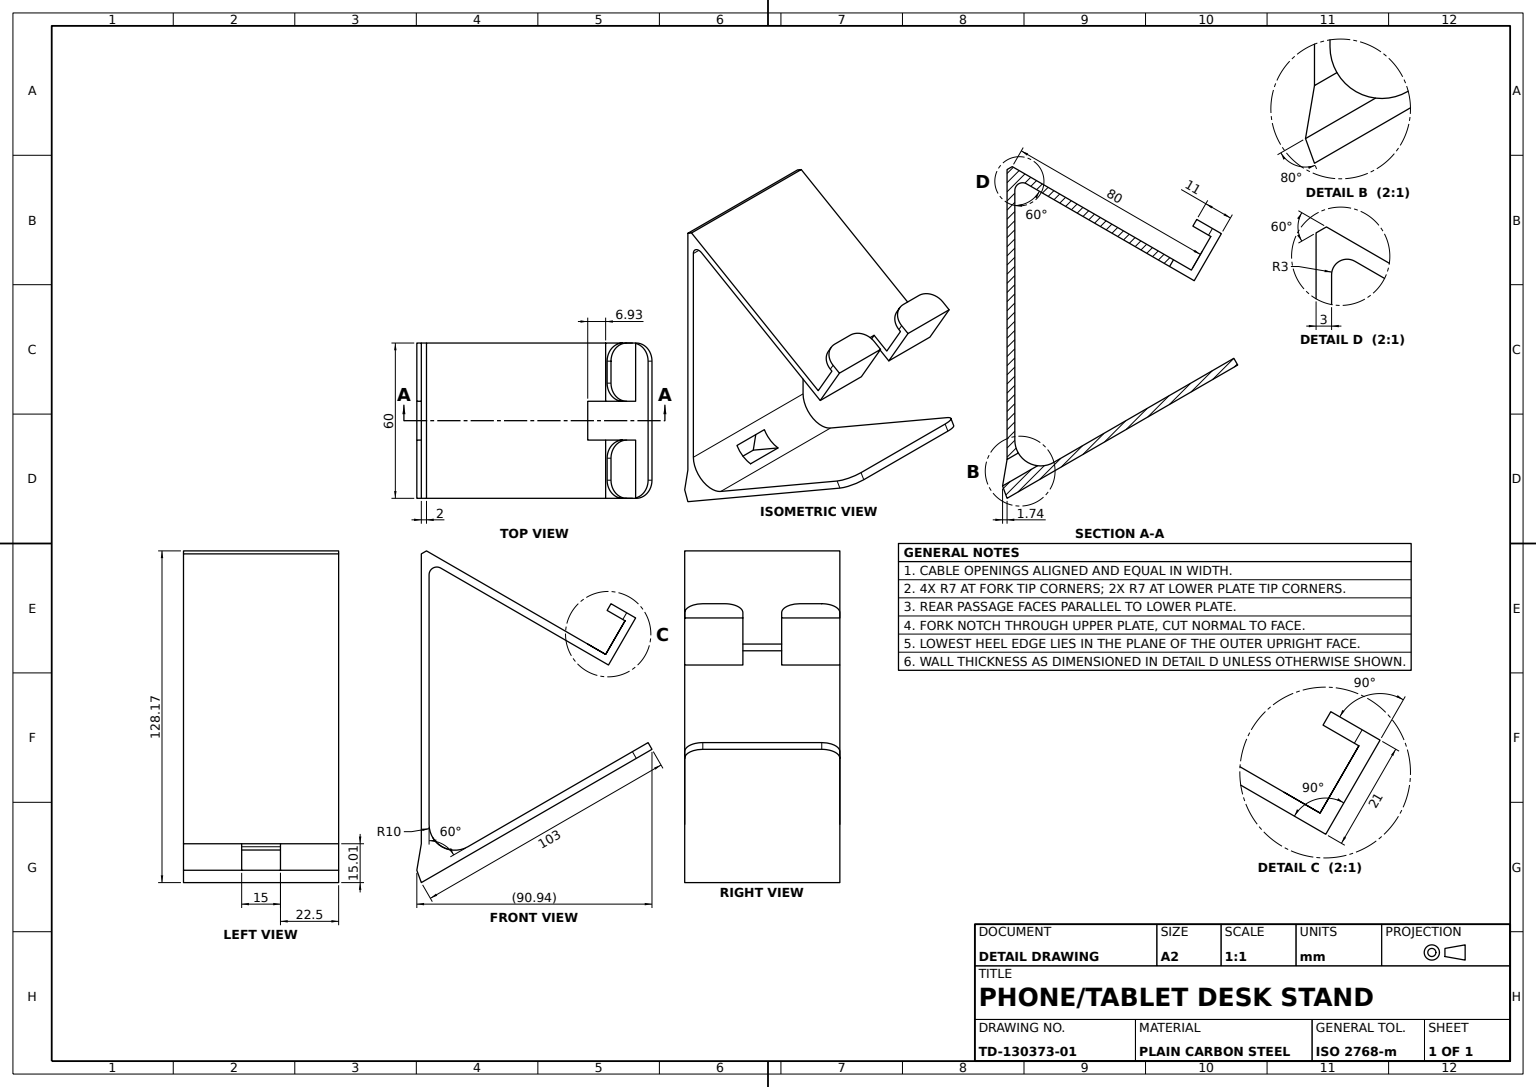
ISO-10303-21;
HEADER;
FILE_DESCRIPTION((''),'2;1');
FILE_NAME('','',(''),(''),'','','');
FILE_SCHEMA(('AUTOMOTIVE_DESIGN'));
ENDSEC;
DATA;
#1=APPLICATION_CONTEXT('');
#2=PRODUCT_CONTEXT('',#1,'mechanical');
#3=PRODUCT('','','',(#2));
#4=PRODUCT_DEFINITION_FORMATION('','',#3);
#5=PRODUCT_DEFINITION_CONTEXT('',#1,'design');
#6=PRODUCT_DEFINITION('','',#4,#5);
#7=PRODUCT_DEFINITION_SHAPE('','',#6);
#8=(LENGTH_UNIT()NAMED_UNIT(*)SI_UNIT(.MILLI.,.METRE.));
#9=(NAMED_UNIT(*)PLANE_ANGLE_UNIT()SI_UNIT($,.RADIAN.));
#10=(NAMED_UNIT(*)SI_UNIT($,.STERADIAN.)SOLID_ANGLE_UNIT());
#11=UNCERTAINTY_MEASURE_WITH_UNIT(LENGTH_MEASURE(1.E-05),#8,'distance_accuracy_value','');
#12=(GEOMETRIC_REPRESENTATION_CONTEXT(3)GLOBAL_UNCERTAINTY_ASSIGNED_CONTEXT((#11))GLOBAL_UNIT_ASSIGNED_CONTEXT((#8,#9,#10))REPRESENTATION_CONTEXT('',''));
#13=CARTESIAN_POINT('',(102.118365,2.,-7.5));
#14=VERTEX_POINT('',#13);
#15=CARTESIAN_POINT('',(86.48334,2.,-7.5));
#16=VERTEX_POINT('',#15);
#17=CARTESIAN_POINT('',(103.,2.,-7.5));
#18=DIRECTION('',(-1.,0.,0.));
#19=VECTOR('',#18,1000.);
#20=LINE('',#17,#19);
#21=EDGE_CURVE('',#14,#16,#20,.T.);
#22=ORIENTED_EDGE('',*,*,#21,.F.);
#23=CARTESIAN_POINT('',(95.494447,10.,-7.5));
#24=VERTEX_POINT('',#23);
#25=DIRECTION('',(-0.637752207,0.7702416,0.));
#26=VECTOR('',#25,1000.);
#27=LINE('',#23,#26);
#28=EDGE_CURVE('',#14,#24,#27,.T.);
#29=ORIENTED_EDGE('',*,*,#28,.T.);
#30=CARTESIAN_POINT('',(90.48334,10.,-7.5));
#31=VERTEX_POINT('',#30);
#32=CARTESIAN_POINT('',(103.,10.,-7.5));
#33=LINE('',#32,#19);
#34=EDGE_CURVE('',#24,#31,#33,.T.);
#35=ORIENTED_EDGE('',*,*,#34,.T.);
#36=CARTESIAN_POINT('',(80.48334,10.,-7.5));
#37=DIRECTION('',(0.,0.,-1.));
#38=DIRECTION('',(1.,0.,0.));
#39=AXIS2_PLACEMENT_3D('',#36,#37,#38);
#40=CIRCLE('',#39,10.);
#41=EDGE_CURVE('',#31,#16,#40,.T.);
#42=ORIENTED_EDGE('',*,*,#41,.T.);
#43=EDGE_LOOP('',(#22,#29,#35,#42));
#44=FACE_OUTER_BOUND('',#43,.T.);
#45=DIRECTION('',(0.,0.,1.));
#46=AXIS2_PLACEMENT_3D('',#17,#45,#38);
#47=PLANE('',#46);
#48=ADVANCED_FACE('',(#44),#47,.T.);
#49=CARTESIAN_POINT('',(-14.406388,53.646171,-23.));
#50=VERTEX_POINT('',#49);
#51=CARTESIAN_POINT('',(-17.906388,47.583993,-30.));
#52=VERTEX_POINT('',#51);
#53=CARTESIAN_POINT('',(-17.906388,47.583993,-23.));
#54=DIRECTION('',(-0.866025404,0.5,0.));
#55=DIRECTION('',(0.5,0.866025404,0.));
#56=AXIS2_PLACEMENT_3D('',#53,#54,#55);
#57=CIRCLE('',#56,7.);
#58=EDGE_CURVE('',#50,#52,#57,.T.);
#59=ORIENTED_EDGE('',*,*,#58,.F.);
#60=CARTESIAN_POINT('',(-11.808312,52.146171,-23.));
#61=VERTEX_POINT('',#60);
#62=VECTOR('',#54,1000.);
#63=LINE('',#49,#62);
#64=EDGE_CURVE('',#61,#50,#63,.T.);
#65=ORIENTED_EDGE('',*,*,#64,.F.);
#66=CARTESIAN_POINT('',(-15.308312,46.083993,-30.));
#67=VERTEX_POINT('',#66);
#68=CARTESIAN_POINT('',(-15.308312,46.083993,-23.));
#69=DIRECTION('',(0.866025404,-0.5,0.));
#70=DIRECTION('',(-0.5,-0.866025404,0.));
#71=AXIS2_PLACEMENT_3D('',#68,#69,#70);
#72=CIRCLE('',#71,7.);
#73=EDGE_CURVE('',#67,#61,#72,.T.);
#74=ORIENTED_EDGE('',*,*,#73,.F.);
#75=CARTESIAN_POINT('',(2.878222,35.583993,-30.));
#76=VECTOR('',#69,1000.);
#77=LINE('',#75,#76);
#78=EDGE_CURVE('',#52,#67,#77,.T.);
#79=ORIENTED_EDGE('',*,*,#78,.F.);
#80=EDGE_LOOP('',(#59,#65,#74,#79));
#81=FACE_OUTER_BOUND('',#80,.T.);
#82=AXIS2_PLACEMENT_3D('',#53,#54,#70);
#83=CYLINDRICAL_SURFACE('',#82,7.);
#84=ADVANCED_FACE('',(#81),#83,.T.);
#85=CARTESIAN_POINT('',(0.,0.,23.));
#86=VERTEX_POINT('',#85);
#87=CARTESIAN_POINT('',(7.,0.,30.));
#88=VERTEX_POINT('',#87);
#89=CARTESIAN_POINT('',(7.,0.,23.));
#90=DIRECTION('',(0.,1.,0.));
#91=AXIS2_PLACEMENT_3D('',#89,#90,#37);
#92=CIRCLE('',#91,7.);
#93=EDGE_CURVE('',#86,#88,#92,.T.);
#94=ORIENTED_EDGE('',*,*,#93,.F.);
#95=CARTESIAN_POINT('',(0.,-3.,23.));
#96=VERTEX_POINT('',#95);
#97=VECTOR('',#90,1000.);
#98=LINE('',#85,#97);
#99=EDGE_CURVE('',#96,#86,#98,.T.);
#100=ORIENTED_EDGE('',*,*,#99,.F.);
#101=CARTESIAN_POINT('',(7.,-3.,30.));
#102=VERTEX_POINT('',#101);
#103=CARTESIAN_POINT('',(7.,-3.,23.));
#104=DIRECTION('',(0.,-1.,0.));
#105=AXIS2_PLACEMENT_3D('',#103,#104,#18);
#106=CIRCLE('',#105,7.);
#107=EDGE_CURVE('',#102,#96,#106,.T.);
#108=ORIENTED_EDGE('',*,*,#107,.F.);
#109=VECTOR('',#104,1000.);
#110=LINE('',#101,#109);
#111=EDGE_CURVE('',#88,#102,#110,.T.);
#112=ORIENTED_EDGE('',*,*,#111,.F.);
#113=EDGE_LOOP('',(#94,#100,#108,#112));
#114=FACE_OUTER_BOUND('',#113,.T.);
#115=CARTESIAN_POINT('',(7.,97.,23.));
#116=AXIS2_PLACEMENT_3D('',#115,#90,#45);
#117=CYLINDRICAL_SURFACE('',#116,7.);
#118=ADVANCED_FACE('',(#114),#117,.T.);
#119=CARTESIAN_POINT('',(103.,-3.,30.));
#120=VERTEX_POINT('',#119);
#121=CARTESIAN_POINT('',(102.118365,2.,30.));
#122=VERTEX_POINT('',#121);
#123=DIRECTION('',(-0.173648178,0.984807753,0.));
#124=VECTOR('',#123,1000.);
#125=LINE('',#119,#124);
#126=EDGE_CURVE('',#120,#122,#125,.T.);
#127=ORIENTED_EDGE('',*,*,#126,.F.);
#128=CARTESIAN_POINT('',(103.,-3.,-30.));
#129=VERTEX_POINT('',#128);
#130=VECTOR('',#37,1000.);
#131=LINE('',#119,#130);
#132=EDGE_CURVE('',#120,#129,#131,.T.);
#133=ORIENTED_EDGE('',*,*,#132,.T.);
#134=CARTESIAN_POINT('',(102.118365,2.,-30.));
#135=VERTEX_POINT('',#134);
#136=LINE('',#128,#124);
#137=EDGE_CURVE('',#129,#135,#136,.T.);
#138=ORIENTED_EDGE('',*,*,#137,.T.);
#139=LINE('',#121,#130);
#140=EDGE_CURVE('',#14,#135,#139,.T.);
#141=ORIENTED_EDGE('',*,*,#140,.F.);
#142=CARTESIAN_POINT('',(102.118365,2.,7.5));
#143=VERTEX_POINT('',#142);
#144=EDGE_CURVE('',#143,#14,#139,.T.);
#145=ORIENTED_EDGE('',*,*,#144,.F.);
#146=EDGE_CURVE('',#122,#143,#139,.T.);
#147=ORIENTED_EDGE('',*,*,#146,.F.);
#148=EDGE_LOOP('',(#127,#133,#138,#141,#145,#147));
#149=FACE_OUTER_BOUND('',#148,.T.);
#150=DIRECTION('',(-0.984807753,-0.173648178,0.));
#151=DIRECTION('',(0.173648178,-0.984807753,0.));
#152=AXIS2_PLACEMENT_3D('',#119,#150,#151);
#153=PLANE('',#152);
#154=ADVANCED_FACE('',(#149),#153,.F.);
#155=CARTESIAN_POINT('',(39.49147,107.,30.));
#156=VERTEX_POINT('',#155);
#157=CARTESIAN_POINT('',(37.182069,107.,30.));
#158=VERTEX_POINT('',#157);
#159=LINE('',#157,#19);
#160=EDGE_CURVE('',#156,#158,#159,.T.);
#161=ORIENTED_EDGE('',*,*,#160,.F.);
#162=CARTESIAN_POINT('',(39.49147,107.,-30.));
#163=VERTEX_POINT('',#162);
#164=LINE('',#155,#130);
#165=EDGE_CURVE('',#156,#163,#164,.T.);
#166=ORIENTED_EDGE('',*,*,#165,.T.);
#167=CARTESIAN_POINT('',(37.182069,107.,-30.));
#168=VERTEX_POINT('',#167);
#169=LINE('',#167,#19);
#170=EDGE_CURVE('',#163,#168,#169,.T.);
#171=ORIENTED_EDGE('',*,*,#170,.T.);
#172=LINE('',#157,#130);
#173=EDGE_CURVE('',#158,#168,#172,.T.);
#174=ORIENTED_EDGE('',*,*,#173,.F.);
#175=EDGE_LOOP('',(#161,#166,#171,#174));
#176=FACE_OUTER_BOUND('',#175,.T.);
#177=AXIS2_PLACEMENT_3D('',#157,#104,#37);
#178=PLANE('',#177);
#179=ADVANCED_FACE('',(#176),#178,.F.);
#180=CARTESIAN_POINT('',(95.494447,10.,7.5));
#181=VERTEX_POINT('',#180);
#182=CARTESIAN_POINT('',(95.494447,10.,30.));
#183=VECTOR('',#45,1000.);
#184=LINE('',#182,#183);
#185=EDGE_CURVE('',#24,#181,#184,.T.);
#186=ORIENTED_EDGE('',*,*,#185,.F.);
#187=CARTESIAN_POINT('',(95.494447,10.,-30.));
#188=VERTEX_POINT('',#187);
#189=LINE('',#182,#130);
#190=EDGE_CURVE('',#24,#188,#189,.T.);
#191=ORIENTED_EDGE('',*,*,#190,.T.);
#192=DIRECTION('',(-0.5,0.866025404,0.));
#193=VECTOR('',#192,1000.);
#194=LINE('',#187,#193);
#195=EDGE_CURVE('',#188,#163,#194,.T.);
#196=ORIENTED_EDGE('',*,*,#195,.T.);
#197=ORIENTED_EDGE('',*,*,#165,.F.);
#198=VERTEX_POINT('',#182);
#199=LINE('',#182,#193);
#200=EDGE_CURVE('',#198,#156,#199,.T.);
#201=ORIENTED_EDGE('',*,*,#200,.F.);
#202=EDGE_CURVE('',#198,#181,#189,.T.);
#203=ORIENTED_EDGE('',*,*,#202,.T.);
#204=EDGE_LOOP('',(#186,#191,#196,#197,#201,#203));
#205=FACE_OUTER_BOUND('',#204,.T.);
#206=DIRECTION('',(-0.866025404,-0.5,0.));
#207=DIRECTION('',(0.5,-0.866025404,0.));
#208=AXIS2_PLACEMENT_3D('',#182,#206,#207);
#209=PLANE('',#208);
#210=ADVANCED_FACE('',(#205),#209,.F.);
#211=CARTESIAN_POINT('',(-1.719854,33.619891,-7.5));
#212=VERTEX_POINT('',#211);
#213=CARTESIAN_POINT('',(-19.906388,44.119891,-7.5));
#214=VERTEX_POINT('',#213);
#215=CARTESIAN_POINT('',(92.678098,-20.880792,-7.5));
#216=LINE('',#215,#62);
#217=EDGE_CURVE('',#212,#214,#216,.T.);
#218=ORIENTED_EDGE('',*,*,#217,.F.);
#219=CARTESIAN_POINT('',(3.780146,43.146171,-7.5));
#220=VERTEX_POINT('',#219);
#221=VECTOR('',#55,1000.);
#222=LINE('',#211,#221);
#223=EDGE_CURVE('',#212,#220,#222,.T.);
#224=ORIENTED_EDGE('',*,*,#223,.T.);
#225=CARTESIAN_POINT('',(1.182069,44.646171,-7.5));
#226=VERTEX_POINT('',#225);
#227=CARTESIAN_POINT('',(98.178098,-11.354512,-7.5));
#228=LINE('',#227,#62);
#229=EDGE_CURVE('',#220,#226,#228,.T.);
#230=ORIENTED_EDGE('',*,*,#229,.T.);
#231=CARTESIAN_POINT('',(-2.817931,37.717968,-7.5));
#232=VERTEX_POINT('',#231);
#233=CARTESIAN_POINT('',(-4.317931,35.119891,-7.5));
#234=VECTOR('',#70,1000.);
#235=LINE('',#233,#234);
#236=EDGE_CURVE('',#226,#232,#235,.T.);
#237=ORIENTED_EDGE('',*,*,#236,.T.);
#238=CARTESIAN_POINT('',(-15.808312,45.217968,-7.5));
#239=VERTEX_POINT('',#238);
#240=CARTESIAN_POINT('',(94.178098,-18.282715,-7.5));
#241=LINE('',#240,#62);
#242=EDGE_CURVE('',#232,#239,#241,.T.);
#243=ORIENTED_EDGE('',*,*,#242,.T.);
#244=CARTESIAN_POINT('',(-15.308312,46.083993,-7.5));
#245=VERTEX_POINT('',#244);
#246=CARTESIAN_POINT('',(-17.308312,42.619891,-7.5));
#247=LINE('',#246,#221);
#248=EDGE_CURVE('',#239,#245,#247,.T.);
#249=ORIENTED_EDGE('',*,*,#248,.T.);
#250=CARTESIAN_POINT('',(-17.906388,47.583993,-7.5));
#251=VERTEX_POINT('',#250);
#252=CARTESIAN_POINT('',(94.678098,-17.41669,-7.5));
#253=LINE('',#252,#62);
#254=EDGE_CURVE('',#245,#251,#253,.T.);
#255=ORIENTED_EDGE('',*,*,#254,.T.);
#256=LINE('',#213,#234);
#257=EDGE_CURVE('',#251,#214,#256,.T.);
#258=ORIENTED_EDGE('',*,*,#257,.T.);
#259=EDGE_LOOP('',(#218,#224,#230,#237,#243,#249,#255,#258));
#260=FACE_OUTER_BOUND('',#259,.T.);
#261=AXIS2_PLACEMENT_3D('',#215,#37,#18);
#262=PLANE('',#261);
#263=ADVANCED_FACE('',(#260),#262,.F.);
#264=CARTESIAN_POINT('',(-19.906388,44.119891,-30.));
#265=VERTEX_POINT('',#264);
#266=LINE('',#264,#234);
#267=EDGE_CURVE('',#52,#265,#266,.T.);
#268=ORIENTED_EDGE('',*,*,#267,.T.);
#269=CARTESIAN_POINT('',(-19.906388,44.119891,30.));
#270=LINE('',#269,#130);
#271=EDGE_CURVE('',#214,#265,#270,.T.);
#272=ORIENTED_EDGE('',*,*,#271,.F.);
#273=ORIENTED_EDGE('',*,*,#257,.F.);
#274=CARTESIAN_POINT('',(-14.406388,53.646171,-14.5));
#275=VERTEX_POINT('',#274);
#276=CARTESIAN_POINT('',(-17.906388,47.583993,-14.5));
#277=AXIS2_PLACEMENT_3D('',#276,#54,#55);
#278=CIRCLE('',#277,7.);
#279=EDGE_CURVE('',#251,#275,#278,.T.);
#280=ORIENTED_EDGE('',*,*,#279,.T.);
#281=CARTESIAN_POINT('',(-14.406388,53.646171,30.));
#282=LINE('',#281,#130);
#283=EDGE_CURVE('',#275,#50,#282,.T.);
#284=ORIENTED_EDGE('',*,*,#283,.T.);
#285=ORIENTED_EDGE('',*,*,#58,.T.);
#286=EDGE_LOOP('',(#268,#272,#273,#280,#284,#285));
#287=FACE_OUTER_BOUND('',#286,.T.);
#288=AXIS2_PLACEMENT_3D('',#269,#69,#55);
#289=PLANE('',#288);
#290=ADVANCED_FACE('',(#287),#289,.F.);
#291=ORIENTED_EDGE('',*,*,#254,.F.);
#292=CARTESIAN_POINT('',(-11.808312,52.146171,-14.5));
#293=VERTEX_POINT('',#292);
#294=CARTESIAN_POINT('',(-15.308312,46.083993,-14.5));
#295=AXIS2_PLACEMENT_3D('',#294,#69,#70);
#296=CIRCLE('',#295,7.);
#297=EDGE_CURVE('',#293,#245,#296,.T.);
#298=ORIENTED_EDGE('',*,*,#297,.F.);
#299=LINE('',#274,#76);
#300=EDGE_CURVE('',#275,#293,#299,.T.);
#301=ORIENTED_EDGE('',*,*,#300,.F.);
#302=ORIENTED_EDGE('',*,*,#279,.F.);
#303=EDGE_LOOP('',(#291,#298,#301,#302));
#304=FACE_OUTER_BOUND('',#303,.T.);
#305=CARTESIAN_POINT('',(94.678098,-17.41669,-14.5));
#306=AXIS2_PLACEMENT_3D('',#305,#54,#70);
#307=CYLINDRICAL_SURFACE('',#306,7.);
#308=ADVANCED_FACE('',(#304),#307,.T.);
#309=CARTESIAN_POINT('',(-14.406388,53.646171,14.5));
#310=VERTEX_POINT('',#309);
#311=CARTESIAN_POINT('',(-17.906388,47.583993,7.5));
#312=VERTEX_POINT('',#311);
#313=CARTESIAN_POINT('',(-17.906388,47.583993,14.5));
#314=AXIS2_PLACEMENT_3D('',#313,#54,#55);
#315=CIRCLE('',#314,7.);
#316=EDGE_CURVE('',#310,#312,#315,.T.);
#317=ORIENTED_EDGE('',*,*,#316,.F.);
#318=CARTESIAN_POINT('',(-11.808312,52.146171,14.5));
#319=VERTEX_POINT('',#318);
#320=LINE('',#309,#62);
#321=EDGE_CURVE('',#319,#310,#320,.T.);
#322=ORIENTED_EDGE('',*,*,#321,.F.);
#323=CARTESIAN_POINT('',(-15.308312,46.083993,7.5));
#324=VERTEX_POINT('',#323);
#325=CARTESIAN_POINT('',(-15.308312,46.083993,14.5));
#326=AXIS2_PLACEMENT_3D('',#325,#69,#70);
#327=CIRCLE('',#326,7.);
#328=EDGE_CURVE('',#324,#319,#327,.T.);
#329=ORIENTED_EDGE('',*,*,#328,.F.);
#330=CARTESIAN_POINT('',(94.678098,-17.41669,7.5));
#331=LINE('',#330,#76);
#332=EDGE_CURVE('',#312,#324,#331,.T.);
#333=ORIENTED_EDGE('',*,*,#332,.F.);
#334=EDGE_LOOP('',(#317,#322,#329,#333));
#335=FACE_OUTER_BOUND('',#334,.T.);
#336=AXIS2_PLACEMENT_3D('',#313,#54,#70);
#337=CYLINDRICAL_SURFACE('',#336,7.);
#338=ADVANCED_FACE('',(#335),#337,.T.);
#339=CARTESIAN_POINT('',(3.780146,43.146171,7.5));
#340=VERTEX_POINT('',#339);
#341=CARTESIAN_POINT('',(-1.719854,33.619891,7.5));
#342=VERTEX_POINT('',#341);
#343=LINE('',#341,#234);
#344=EDGE_CURVE('',#340,#342,#343,.T.);
#345=ORIENTED_EDGE('',*,*,#344,.F.);
#346=LINE('',#219,#183);
#347=EDGE_CURVE('',#220,#340,#346,.T.);
#348=ORIENTED_EDGE('',*,*,#347,.F.);
#349=ORIENTED_EDGE('',*,*,#223,.F.);
#350=CARTESIAN_POINT('',(-1.719854,33.619891,-30.));
#351=VERTEX_POINT('',#350);
#352=CARTESIAN_POINT('',(-1.719854,33.619891,30.));
#353=LINE('',#352,#130);
#354=EDGE_CURVE('',#212,#351,#353,.T.);
#355=ORIENTED_EDGE('',*,*,#354,.T.);
#356=CARTESIAN_POINT('',(35.738694,98.5,-30.));
#357=VERTEX_POINT('',#356);
#358=LINE('',#356,#221);
#359=EDGE_CURVE('',#351,#357,#358,.T.);
#360=ORIENTED_EDGE('',*,*,#359,.T.);
#361=CARTESIAN_POINT('',(35.738694,98.5,30.));
#362=VERTEX_POINT('',#361);
#363=LINE('',#361,#130);
#364=EDGE_CURVE('',#362,#357,#363,.T.);
#365=ORIENTED_EDGE('',*,*,#364,.F.);
#366=VERTEX_POINT('',#352);
#367=LINE('',#361,#221);
#368=EDGE_CURVE('',#366,#362,#367,.T.);
#369=ORIENTED_EDGE('',*,*,#368,.F.);
#370=EDGE_CURVE('',#366,#342,#353,.T.);
#371=ORIENTED_EDGE('',*,*,#370,.T.);
#372=EDGE_LOOP('',(#345,#348,#349,#355,#360,#365,#369,#371));
#373=FACE_OUTER_BOUND('',#372,.T.);
#374=AXIS2_PLACEMENT_3D('',#361,#54,#70);
#375=PLANE('',#374);
#376=ADVANCED_FACE('',(#373),#375,.F.);
#377=CARTESIAN_POINT('',(-17.906388,47.583993,30.));
#378=VERTEX_POINT('',#377);
#379=VERTEX_POINT('',#269);
#380=LINE('',#269,#234);
#381=EDGE_CURVE('',#378,#379,#380,.T.);
#382=ORIENTED_EDGE('',*,*,#381,.F.);
#383=CARTESIAN_POINT('',(-14.406388,53.646171,23.));
#384=VERTEX_POINT('',#383);
#385=CARTESIAN_POINT('',(-17.906388,47.583993,23.));
#386=AXIS2_PLACEMENT_3D('',#385,#54,#55);
#387=CIRCLE('',#386,7.);
#388=EDGE_CURVE('',#378,#384,#387,.T.);
#389=ORIENTED_EDGE('',*,*,#388,.T.);
#390=EDGE_CURVE('',#384,#310,#282,.T.);
#391=ORIENTED_EDGE('',*,*,#390,.T.);
#392=ORIENTED_EDGE('',*,*,#316,.T.);
#393=CARTESIAN_POINT('',(-19.906388,44.119891,7.5));
#394=VERTEX_POINT('',#393);
#395=LINE('',#393,#221);
#396=EDGE_CURVE('',#394,#312,#395,.T.);
#397=ORIENTED_EDGE('',*,*,#396,.F.);
#398=EDGE_CURVE('',#379,#394,#270,.T.);
#399=ORIENTED_EDGE('',*,*,#398,.F.);
#400=EDGE_LOOP('',(#382,#389,#391,#392,#397,#399));
#401=FACE_OUTER_BOUND('',#400,.T.);
#402=ADVANCED_FACE('',(#401),#289,.F.);
#403=LINE('',#187,#26);
#404=EDGE_CURVE('',#135,#188,#403,.T.);
#405=ORIENTED_EDGE('',*,*,#404,.T.);
#406=ORIENTED_EDGE('',*,*,#190,.F.);
#407=ORIENTED_EDGE('',*,*,#28,.F.);
#408=ORIENTED_EDGE('',*,*,#140,.T.);
#409=EDGE_LOOP('',(#405,#406,#407,#408));
#410=FACE_OUTER_BOUND('',#409,.T.);
#411=DIRECTION('',(-0.7702416,-0.637752207,0.));
#412=DIRECTION('',(0.637752207,-0.7702416,0.));
#413=AXIS2_PLACEMENT_3D('',#182,#411,#412);
#414=PLANE('',#413);
#415=ADVANCED_FACE('',(#410),#414,.F.);
#416=CARTESIAN_POINT('',(-11.808312,52.146171,23.));
#417=VERTEX_POINT('',#416);
#418=CARTESIAN_POINT('',(-15.308312,46.083993,30.));
#419=VERTEX_POINT('',#418);
#420=CARTESIAN_POINT('',(-15.308312,46.083993,23.));
#421=AXIS2_PLACEMENT_3D('',#420,#69,#70);
#422=CIRCLE('',#421,7.);
#423=EDGE_CURVE('',#417,#419,#422,.T.);
#424=ORIENTED_EDGE('',*,*,#423,.T.);
#425=CARTESIAN_POINT('',(-15.808312,45.217968,30.));
#426=VERTEX_POINT('',#425);
#427=LINE('',#425,#221);
#428=EDGE_CURVE('',#426,#419,#427,.T.);
#429=ORIENTED_EDGE('',*,*,#428,.F.);
#430=CARTESIAN_POINT('',(-15.808312,45.217968,7.5));
#431=VERTEX_POINT('',#430);
#432=LINE('',#425,#130);
#433=EDGE_CURVE('',#426,#431,#432,.T.);
#434=ORIENTED_EDGE('',*,*,#433,.T.);
#435=CARTESIAN_POINT('',(-17.308312,42.619891,7.5));
#436=LINE('',#435,#234);
#437=EDGE_CURVE('',#324,#431,#436,.T.);
#438=ORIENTED_EDGE('',*,*,#437,.F.);
#439=ORIENTED_EDGE('',*,*,#328,.T.);
#440=CARTESIAN_POINT('',(-11.808312,52.146171,30.));
#441=LINE('',#440,#130);
#442=EDGE_CURVE('',#417,#319,#441,.T.);
#443=ORIENTED_EDGE('',*,*,#442,.F.);
#444=EDGE_LOOP('',(#424,#429,#434,#438,#439,#443));
#445=FACE_OUTER_BOUND('',#444,.T.);
#446=AXIS2_PLACEMENT_3D('',#425,#54,#70);
#447=PLANE('',#446);
#448=ADVANCED_FACE('',(#445),#447,.F.);
#449=CARTESIAN_POINT('',(-2.817931,37.717968,30.));
#450=VERTEX_POINT('',#449);
#451=CARTESIAN_POINT('',(-2.817931,37.717968,7.5));
#452=VERTEX_POINT('',#451);
#453=LINE('',#449,#130);
#454=EDGE_CURVE('',#450,#452,#453,.T.);
#455=ORIENTED_EDGE('',*,*,#454,.T.);
#456=CARTESIAN_POINT('',(94.178098,-18.282715,7.5));
#457=LINE('',#456,#76);
#458=EDGE_CURVE('',#431,#452,#457,.T.);
#459=ORIENTED_EDGE('',*,*,#458,.F.);
#460=ORIENTED_EDGE('',*,*,#433,.F.);
#461=LINE('',#449,#62);
#462=EDGE_CURVE('',#450,#426,#461,.T.);
#463=ORIENTED_EDGE('',*,*,#462,.F.);
#464=EDGE_LOOP('',(#455,#459,#460,#463));
#465=FACE_OUTER_BOUND('',#464,.T.);
#466=AXIS2_PLACEMENT_3D('',#449,#70,#69);
#467=PLANE('',#466);
#468=ADVANCED_FACE('',(#465),#467,.F.);
#469=CARTESIAN_POINT('',(86.48334,2.,7.5));
#470=VERTEX_POINT('',#469);
#471=CARTESIAN_POINT('',(103.,2.,7.5));
#472=LINE('',#471,#19);
#473=EDGE_CURVE('',#143,#470,#472,.T.);
#474=ORIENTED_EDGE('',*,*,#473,.T.);
#475=CARTESIAN_POINT('',(90.48334,10.,7.5));
#476=VERTEX_POINT('',#475);
#477=CARTESIAN_POINT('',(80.48334,10.,7.5));
#478=AXIS2_PLACEMENT_3D('',#477,#45,#18);
#479=CIRCLE('',#478,10.);
#480=EDGE_CURVE('',#470,#476,#479,.T.);
#481=ORIENTED_EDGE('',*,*,#480,.T.);
#482=CARTESIAN_POINT('',(103.,10.,7.5));
#483=LINE('',#482,#19);
#484=EDGE_CURVE('',#181,#476,#483,.T.);
#485=ORIENTED_EDGE('',*,*,#484,.F.);
#486=VECTOR('',#412,1000.);
#487=LINE('',#180,#486);
#488=EDGE_CURVE('',#181,#143,#487,.T.);
#489=ORIENTED_EDGE('',*,*,#488,.T.);
#490=EDGE_LOOP('',(#474,#481,#485,#489));
#491=FACE_OUTER_BOUND('',#490,.T.);
#492=AXIS2_PLACEMENT_3D('',#471,#37,#18);
#493=PLANE('',#492);
#494=ADVANCED_FACE('',(#491),#493,.T.);
#495=ORIENTED_EDGE('',*,*,#242,.F.);
#496=CARTESIAN_POINT('',(-2.817931,37.717968,-30.));
#497=VERTEX_POINT('',#496);
#498=EDGE_CURVE('',#232,#497,#453,.T.);
#499=ORIENTED_EDGE('',*,*,#498,.T.);
#500=CARTESIAN_POINT('',(-15.808312,45.217968,-30.));
#501=VERTEX_POINT('',#500);
#502=LINE('',#496,#62);
#503=EDGE_CURVE('',#497,#501,#502,.T.);
#504=ORIENTED_EDGE('',*,*,#503,.T.);
#505=EDGE_CURVE('',#239,#501,#432,.T.);
#506=ORIENTED_EDGE('',*,*,#505,.F.);
#507=EDGE_LOOP('',(#495,#499,#504,#506));
#508=FACE_OUTER_BOUND('',#507,.T.);
#509=ADVANCED_FACE('',(#508),#467,.F.);
#510=ORIENTED_EDGE('',*,*,#107,.T.);
#511=CARTESIAN_POINT('',(0.,-3.,-23.));
#512=VERTEX_POINT('',#511);
#513=CARTESIAN_POINT('',(0.,-3.,30.));
#514=LINE('',#513,#130);
#515=EDGE_CURVE('',#96,#512,#514,.T.);
#516=ORIENTED_EDGE('',*,*,#515,.T.);
#517=CARTESIAN_POINT('',(7.,-3.,-30.));
#518=VERTEX_POINT('',#517);
#519=CARTESIAN_POINT('',(7.,-3.,-23.));
#520=AXIS2_PLACEMENT_3D('',#519,#104,#18);
#521=CIRCLE('',#520,7.);
#522=EDGE_CURVE('',#512,#518,#521,.T.);
#523=ORIENTED_EDGE('',*,*,#522,.T.);
#524=CARTESIAN_POINT('',(0.,-3.,-30.));
#525=VECTOR('',#38,1000.);
#526=LINE('',#524,#525);
#527=EDGE_CURVE('',#518,#129,#526,.T.);
#528=ORIENTED_EDGE('',*,*,#527,.T.);
#529=ORIENTED_EDGE('',*,*,#132,.F.);
#530=LINE('',#513,#525);
#531=EDGE_CURVE('',#102,#120,#530,.T.);
#532=ORIENTED_EDGE('',*,*,#531,.F.);
#533=EDGE_LOOP('',(#510,#516,#523,#528,#529,#532));
#534=FACE_OUTER_BOUND('',#533,.T.);
#535=AXIS2_PLACEMENT_3D('',#513,#90,#18);
#536=PLANE('',#535);
#537=ADVANCED_FACE('',(#534),#536,.F.);
#538=ORIENTED_EDGE('',*,*,#185,.T.);
#539=ORIENTED_EDGE('',*,*,#484,.T.);
#540=CARTESIAN_POINT('',(90.48334,10.,30.));
#541=LINE('',#540,#130);
#542=EDGE_CURVE('',#476,#31,#541,.T.);
#543=ORIENTED_EDGE('',*,*,#542,.T.);
#544=ORIENTED_EDGE('',*,*,#34,.F.);
#545=EDGE_LOOP('',(#538,#539,#543,#544));
#546=FACE_OUTER_BOUND('',#545,.T.);
#547=AXIS2_PLACEMENT_3D('',#482,#104,#37);
#548=PLANE('',#547);
#549=ADVANCED_FACE('',(#546),#548,.T.);
#550=ORIENTED_EDGE('',*,*,#283,.F.);
#551=ORIENTED_EDGE('',*,*,#300,.T.);
#552=EDGE_CURVE('',#293,#61,#441,.T.);
#553=ORIENTED_EDGE('',*,*,#552,.T.);
#554=ORIENTED_EDGE('',*,*,#64,.T.);
#555=EDGE_LOOP('',(#550,#551,#553,#554));
#556=FACE_OUTER_BOUND('',#555,.T.);
#557=AXIS2_PLACEMENT_3D('',#281,#70,#69);
#558=PLANE('',#557);
#559=ADVANCED_FACE('',(#556),#558,.F.);
#560=LINE('',#500,#221);
#561=EDGE_CURVE('',#501,#67,#560,.T.);
#562=ORIENTED_EDGE('',*,*,#561,.T.);
#563=ORIENTED_EDGE('',*,*,#73,.T.);
#564=ORIENTED_EDGE('',*,*,#552,.F.);
#565=ORIENTED_EDGE('',*,*,#297,.T.);
#566=ORIENTED_EDGE('',*,*,#248,.F.);
#567=ORIENTED_EDGE('',*,*,#505,.T.);
#568=EDGE_LOOP('',(#562,#563,#564,#565,#566,#567));
#569=FACE_OUTER_BOUND('',#568,.T.);
#570=ADVANCED_FACE('',(#569),#447,.F.);
#571=LINE('',#377,#62);
#572=EDGE_CURVE('',#419,#378,#571,.T.);
#573=ORIENTED_EDGE('',*,*,#572,.T.);
#574=ORIENTED_EDGE('',*,*,#381,.T.);
#575=LINE('',#352,#76);
#576=EDGE_CURVE('',#379,#366,#575,.T.);
#577=ORIENTED_EDGE('',*,*,#576,.T.);
#578=ORIENTED_EDGE('',*,*,#368,.T.);
#579=CARTESIAN_POINT('',(40.934846,98.5,30.));
#580=VERTEX_POINT('',#579);
#581=CARTESIAN_POINT('',(38.33677,97.,30.));
#582=AXIS2_PLACEMENT_3D('',#581,#37,#38);
#583=CIRCLE('',#582,3.);
#584=EDGE_CURVE('',#362,#580,#583,.T.);
#585=ORIENTED_EDGE('',*,*,#584,.T.);
#586=CARTESIAN_POINT('',(89.143594,15.,30.));
#587=VERTEX_POINT('',#586);
#588=VECTOR('',#207,1000.);
#589=LINE('',#586,#588);
#590=EDGE_CURVE('',#580,#587,#589,.T.);
#591=ORIENTED_EDGE('',*,*,#590,.T.);
#592=CARTESIAN_POINT('',(80.48334,0.,30.));
#593=VERTEX_POINT('',#592);
#594=CARTESIAN_POINT('',(80.48334,10.,30.));
#595=AXIS2_PLACEMENT_3D('',#594,#37,#38);
#596=CIRCLE('',#595,10.);
#597=EDGE_CURVE('',#587,#593,#596,.T.);
#598=ORIENTED_EDGE('',*,*,#597,.T.);
#599=CARTESIAN_POINT('',(0.,0.,30.));
#600=LINE('',#599,#19);
#601=EDGE_CURVE('',#593,#88,#600,.T.);
#602=ORIENTED_EDGE('',*,*,#601,.T.);
#603=ORIENTED_EDGE('',*,*,#111,.T.);
#604=ORIENTED_EDGE('',*,*,#531,.T.);
#605=ORIENTED_EDGE('',*,*,#126,.T.);
#606=LINE('',#182,#26);
#607=EDGE_CURVE('',#122,#198,#606,.T.);
#608=ORIENTED_EDGE('',*,*,#607,.T.);
#609=ORIENTED_EDGE('',*,*,#200,.T.);
#610=ORIENTED_EDGE('',*,*,#160,.T.);
#611=LINE('',#157,#234);
#612=EDGE_CURVE('',#158,#450,#611,.T.);
#613=ORIENTED_EDGE('',*,*,#612,.T.);
#614=ORIENTED_EDGE('',*,*,#462,.T.);
#615=ORIENTED_EDGE('',*,*,#428,.T.);
#616=EDGE_LOOP('',(#573,#574,#577,#578,#585,#591,#598,#602,#603,#604,#605,#608,#609,#610,#613,#614,#615));
#617=FACE_OUTER_BOUND('',#616,.T.);
#618=AXIS2_PLACEMENT_3D('',#581,#45,#38);
#619=PLANE('',#618);
#620=ADVANCED_FACE('',(#617),#619,.T.);
#621=ORIENTED_EDGE('',*,*,#576,.F.);
#622=ORIENTED_EDGE('',*,*,#398,.T.);
#623=CARTESIAN_POINT('',(92.678098,-20.880792,7.5));
#624=LINE('',#623,#62);
#625=EDGE_CURVE('',#342,#394,#624,.T.);
#626=ORIENTED_EDGE('',*,*,#625,.F.);
#627=ORIENTED_EDGE('',*,*,#370,.F.);
#628=EDGE_LOOP('',(#621,#622,#626,#627));
#629=FACE_OUTER_BOUND('',#628,.T.);
#630=AXIS2_PLACEMENT_3D('',#352,#55,#54);
#631=PLANE('',#630);
#632=ADVANCED_FACE('',(#629),#631,.F.);
#633=CARTESIAN_POINT('',(40.934846,98.5,-30.));
#634=VERTEX_POINT('',#633);
#635=CARTESIAN_POINT('',(38.33677,97.,-30.));
#636=AXIS2_PLACEMENT_3D('',#635,#37,#38);
#637=CIRCLE('',#636,3.);
#638=EDGE_CURVE('',#357,#634,#637,.T.);
#639=ORIENTED_EDGE('',*,*,#638,.T.);
#640=LINE('',#579,#130);
#641=EDGE_CURVE('',#580,#634,#640,.T.);
#642=ORIENTED_EDGE('',*,*,#641,.F.);
#643=ORIENTED_EDGE('',*,*,#584,.F.);
#644=ORIENTED_EDGE('',*,*,#364,.T.);
#645=EDGE_LOOP('',(#639,#642,#643,#644));
#646=FACE_OUTER_BOUND('',#645,.T.);
#647=AXIS2_PLACEMENT_3D('',#581,#37,#18);
#648=CYLINDRICAL_SURFACE('',#647,3.);
#649=ADVANCED_FACE('',(#646),#648,.F.);
#650=ORIENTED_EDGE('',*,*,#561,.F.);
#651=ORIENTED_EDGE('',*,*,#503,.F.);
#652=LINE('',#167,#234);
#653=EDGE_CURVE('',#168,#497,#652,.T.);
#654=ORIENTED_EDGE('',*,*,#653,.F.);
#655=ORIENTED_EDGE('',*,*,#170,.F.);
#656=ORIENTED_EDGE('',*,*,#195,.F.);
#657=ORIENTED_EDGE('',*,*,#404,.F.);
#658=ORIENTED_EDGE('',*,*,#137,.F.);
#659=ORIENTED_EDGE('',*,*,#527,.F.);
#660=CARTESIAN_POINT('',(7.,0.,-30.));
#661=VERTEX_POINT('',#660);
#662=CARTESIAN_POINT('',(7.,97.,-30.));
#663=LINE('',#662,#97);
#664=EDGE_CURVE('',#518,#661,#663,.T.);
#665=ORIENTED_EDGE('',*,*,#664,.T.);
#666=CARTESIAN_POINT('',(80.48334,0.,-30.));
#667=VERTEX_POINT('',#666);
#668=CARTESIAN_POINT('',(0.,0.,-30.));
#669=LINE('',#668,#19);
#670=EDGE_CURVE('',#667,#661,#669,.T.);
#671=ORIENTED_EDGE('',*,*,#670,.F.);
#672=CARTESIAN_POINT('',(89.143594,15.,-30.));
#673=VERTEX_POINT('',#672);
#674=CARTESIAN_POINT('',(80.48334,10.,-30.));
#675=AXIS2_PLACEMENT_3D('',#674,#37,#38);
#676=CIRCLE('',#675,10.);
#677=EDGE_CURVE('',#673,#667,#676,.T.);
#678=ORIENTED_EDGE('',*,*,#677,.F.);
#679=LINE('',#672,#588);
#680=EDGE_CURVE('',#634,#673,#679,.T.);
#681=ORIENTED_EDGE('',*,*,#680,.F.);
#682=ORIENTED_EDGE('',*,*,#638,.F.);
#683=ORIENTED_EDGE('',*,*,#359,.F.);
#684=LINE('',#350,#76);
#685=EDGE_CURVE('',#265,#351,#684,.T.);
#686=ORIENTED_EDGE('',*,*,#685,.F.);
#687=ORIENTED_EDGE('',*,*,#267,.F.);
#688=ORIENTED_EDGE('',*,*,#78,.T.);
#689=EDGE_LOOP('',(#650,#651,#654,#655,#656,#657,#658,#659,#665,#671,#678,#681,#682,#683,#686,#687,#688));
#690=FACE_OUTER_BOUND('',#689,.T.);
#691=AXIS2_PLACEMENT_3D('',#635,#45,#38);
#692=PLANE('',#691);
#693=ADVANCED_FACE('',(#690),#692,.F.);
#694=CARTESIAN_POINT('',(1.182069,44.646171,7.5));
#695=VERTEX_POINT('',#694);
#696=CARTESIAN_POINT('',(98.178098,-11.354512,7.5));
#697=LINE('',#696,#62);
#698=EDGE_CURVE('',#340,#695,#697,.T.);
#699=ORIENTED_EDGE('',*,*,#698,.T.);
#700=LINE('',#225,#130);
#701=EDGE_CURVE('',#695,#226,#700,.T.);
#702=ORIENTED_EDGE('',*,*,#701,.T.);
#703=ORIENTED_EDGE('',*,*,#229,.F.);
#704=ORIENTED_EDGE('',*,*,#347,.T.);
#705=EDGE_LOOP('',(#699,#702,#703,#704));
#706=FACE_OUTER_BOUND('',#705,.T.);
#707=AXIS2_PLACEMENT_3D('',#227,#55,#54);
#708=PLANE('',#707);
#709=ADVANCED_FACE('',(#706),#708,.F.);
#710=ORIENTED_EDGE('',*,*,#680,.T.);
#711=LINE('',#586,#130);
#712=EDGE_CURVE('',#587,#673,#711,.T.);
#713=ORIENTED_EDGE('',*,*,#712,.F.);
#714=ORIENTED_EDGE('',*,*,#590,.F.);
#715=ORIENTED_EDGE('',*,*,#641,.T.);
#716=EDGE_LOOP('',(#710,#713,#714,#715));
#717=FACE_OUTER_BOUND('',#716,.T.);
#718=DIRECTION('',(0.866025404,0.5,0.));
#719=AXIS2_PLACEMENT_3D('',#586,#718,#192);
#720=PLANE('',#719);
#721=ADVANCED_FACE('',(#717),#720,.F.);
#722=ORIENTED_EDGE('',*,*,#202,.F.);
#723=ORIENTED_EDGE('',*,*,#607,.F.);
#724=ORIENTED_EDGE('',*,*,#146,.T.);
#725=ORIENTED_EDGE('',*,*,#488,.F.);
#726=EDGE_LOOP('',(#722,#723,#724,#725));
#727=FACE_OUTER_BOUND('',#726,.T.);
#728=ADVANCED_FACE('',(#727),#414,.F.);
#729=ORIENTED_EDGE('',*,*,#144,.T.);
#730=ORIENTED_EDGE('',*,*,#21,.T.);
#731=CARTESIAN_POINT('',(86.48334,2.,30.));
#732=LINE('',#731,#183);
#733=EDGE_CURVE('',#16,#470,#732,.T.);
#734=ORIENTED_EDGE('',*,*,#733,.T.);
#735=ORIENTED_EDGE('',*,*,#473,.F.);
#736=EDGE_LOOP('',(#729,#730,#734,#735));
#737=FACE_OUTER_BOUND('',#736,.T.);
#738=AXIS2_PLACEMENT_3D('',#471,#90,#45);
#739=PLANE('',#738);
#740=ADVANCED_FACE('',(#737),#739,.T.);
#741=ORIENTED_EDGE('',*,*,#396,.T.);
#742=ORIENTED_EDGE('',*,*,#332,.T.);
#743=ORIENTED_EDGE('',*,*,#437,.T.);
#744=ORIENTED_EDGE('',*,*,#458,.T.);
#745=CARTESIAN_POINT('',(-4.317931,35.119891,7.5));
#746=LINE('',#745,#221);
#747=EDGE_CURVE('',#452,#695,#746,.T.);
#748=ORIENTED_EDGE('',*,*,#747,.T.);
#749=ORIENTED_EDGE('',*,*,#698,.F.);
#750=ORIENTED_EDGE('',*,*,#344,.T.);
#751=ORIENTED_EDGE('',*,*,#625,.T.);
#752=EDGE_LOOP('',(#741,#742,#743,#744,#748,#749,#750,#751));
#753=FACE_OUTER_BOUND('',#752,.T.);
#754=AXIS2_PLACEMENT_3D('',#623,#45,#38);
#755=PLANE('',#754);
#756=ADVANCED_FACE('',(#753),#755,.F.);
#757=LINE('',#592,#130);
#758=EDGE_CURVE('',#593,#667,#757,.T.);
#759=ORIENTED_EDGE('',*,*,#758,.T.);
#760=ORIENTED_EDGE('',*,*,#670,.T.);
#761=CARTESIAN_POINT('',(0.,0.,-23.));
#762=VERTEX_POINT('',#761);
#763=CARTESIAN_POINT('',(7.,0.,-23.));
#764=AXIS2_PLACEMENT_3D('',#763,#90,#37);
#765=CIRCLE('',#764,7.);
#766=EDGE_CURVE('',#661,#762,#765,.T.);
#767=ORIENTED_EDGE('',*,*,#766,.T.);
#768=LINE('',#599,#130);
#769=EDGE_CURVE('',#86,#762,#768,.T.);
#770=ORIENTED_EDGE('',*,*,#769,.F.);
#771=ORIENTED_EDGE('',*,*,#93,.T.);
#772=ORIENTED_EDGE('',*,*,#601,.F.);
#773=EDGE_LOOP('',(#759,#760,#767,#770,#771,#772));
#774=FACE_OUTER_BOUND('',#773,.T.);
#775=AXIS2_PLACEMENT_3D('',#599,#104,#37);
#776=PLANE('',#775);
#777=ADVANCED_FACE('',(#774),#776,.F.);
#778=ORIENTED_EDGE('',*,*,#664,.F.);
#779=ORIENTED_EDGE('',*,*,#522,.F.);
#780=LINE('',#761,#109);
#781=EDGE_CURVE('',#762,#512,#780,.T.);
#782=ORIENTED_EDGE('',*,*,#781,.F.);
#783=ORIENTED_EDGE('',*,*,#766,.F.);
#784=EDGE_LOOP('',(#778,#779,#782,#783));
#785=FACE_OUTER_BOUND('',#784,.T.);
#786=AXIS2_PLACEMENT_3D('',#763,#104,#37);
#787=CYLINDRICAL_SURFACE('',#786,7.);
#788=ADVANCED_FACE('',(#785),#787,.T.);
#789=ORIENTED_EDGE('',*,*,#442,.T.);
#790=ORIENTED_EDGE('',*,*,#321,.T.);
#791=ORIENTED_EDGE('',*,*,#390,.F.);
#792=LINE('',#416,#76);
#793=EDGE_CURVE('',#384,#417,#792,.T.);
#794=ORIENTED_EDGE('',*,*,#793,.T.);
#795=EDGE_LOOP('',(#789,#790,#791,#794));
#796=FACE_OUTER_BOUND('',#795,.T.);
#797=ADVANCED_FACE('',(#796),#558,.F.);
#798=ORIENTED_EDGE('',*,*,#677,.T.);
#799=ORIENTED_EDGE('',*,*,#758,.F.);
#800=ORIENTED_EDGE('',*,*,#597,.F.);
#801=ORIENTED_EDGE('',*,*,#712,.T.);
#802=EDGE_LOOP('',(#798,#799,#800,#801));
#803=FACE_OUTER_BOUND('',#802,.T.);
#804=ORIENTED_EDGE('',*,*,#41,.F.);
#805=ORIENTED_EDGE('',*,*,#542,.F.);
#806=ORIENTED_EDGE('',*,*,#480,.F.);
#807=ORIENTED_EDGE('',*,*,#733,.F.);
#808=EDGE_LOOP('',(#804,#805,#806,#807));
#809=FACE_BOUND('',#808,.T.);
#810=AXIS2_PLACEMENT_3D('',#594,#37,#18);
#811=CYLINDRICAL_SURFACE('',#810,10.);
#812=ADVANCED_FACE('',(#803,#809),#811,.F.);
#813=ORIENTED_EDGE('',*,*,#701,.F.);
#814=ORIENTED_EDGE('',*,*,#747,.F.);
#815=ORIENTED_EDGE('',*,*,#454,.F.);
#816=ORIENTED_EDGE('',*,*,#612,.F.);
#817=ORIENTED_EDGE('',*,*,#173,.T.);
#818=ORIENTED_EDGE('',*,*,#653,.T.);
#819=ORIENTED_EDGE('',*,*,#498,.F.);
#820=ORIENTED_EDGE('',*,*,#236,.F.);
#821=EDGE_LOOP('',(#813,#814,#815,#816,#817,#818,#819,#820));
#822=FACE_OUTER_BOUND('',#821,.T.);
#823=AXIS2_PLACEMENT_3D('',#157,#69,#55);
#824=PLANE('',#823);
#825=ADVANCED_FACE('',(#822),#824,.F.);
#826=ORIENTED_EDGE('',*,*,#217,.T.);
#827=ORIENTED_EDGE('',*,*,#271,.T.);
#828=ORIENTED_EDGE('',*,*,#685,.T.);
#829=ORIENTED_EDGE('',*,*,#354,.F.);
#830=EDGE_LOOP('',(#826,#827,#828,#829));
#831=FACE_OUTER_BOUND('',#830,.T.);
#832=ADVANCED_FACE('',(#831),#631,.F.);
#833=ORIENTED_EDGE('',*,*,#515,.F.);
#834=ORIENTED_EDGE('',*,*,#99,.T.);
#835=ORIENTED_EDGE('',*,*,#769,.T.);
#836=ORIENTED_EDGE('',*,*,#781,.T.);
#837=EDGE_LOOP('',(#833,#834,#835,#836));
#838=FACE_OUTER_BOUND('',#837,.T.);
#839=AXIS2_PLACEMENT_3D('',#599,#38,#37);
#840=PLANE('',#839);
#841=ADVANCED_FACE('',(#838),#840,.F.);
#842=ORIENTED_EDGE('',*,*,#423,.F.);
#843=ORIENTED_EDGE('',*,*,#793,.F.);
#844=ORIENTED_EDGE('',*,*,#388,.F.);
#845=ORIENTED_EDGE('',*,*,#572,.F.);
#846=EDGE_LOOP('',(#842,#843,#844,#845));
#847=FACE_OUTER_BOUND('',#846,.T.);
#848=CARTESIAN_POINT('',(2.878222,35.583993,23.));
#849=AXIS2_PLACEMENT_3D('',#848,#69,#55);
#850=CYLINDRICAL_SURFACE('',#849,7.);
#851=ADVANCED_FACE('',(#847),#850,.T.);
#852=CLOSED_SHELL('',(#48,#84,#118,#154,#179,#210,#263,#290,#308,#338,#376,#402,#415,#448,#468,#494,#509,#537,#549,#559,#570,#620,#632,#649,#693,#709,#721,#728,#740,#756,#777,#788,#797,#812,#825,#832,#841,#851));
#853=MANIFOLD_SOLID_BREP('',#852);
#854=ADVANCED_BREP_SHAPE_REPRESENTATION('',(#853),#12);
#855=SHAPE_DEFINITION_REPRESENTATION(#7,#854);
ENDSEC;
END-ISO-10303-21;
